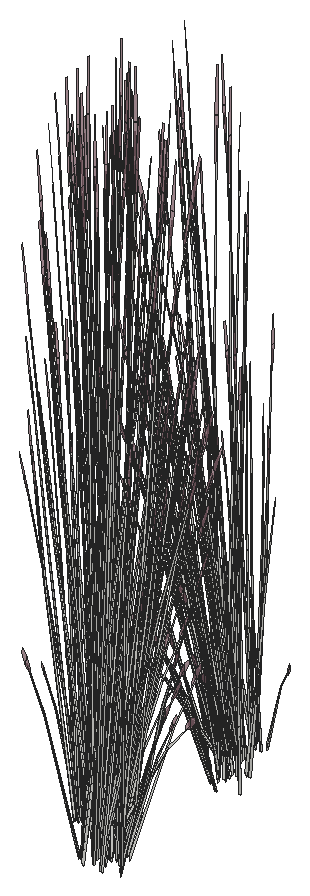
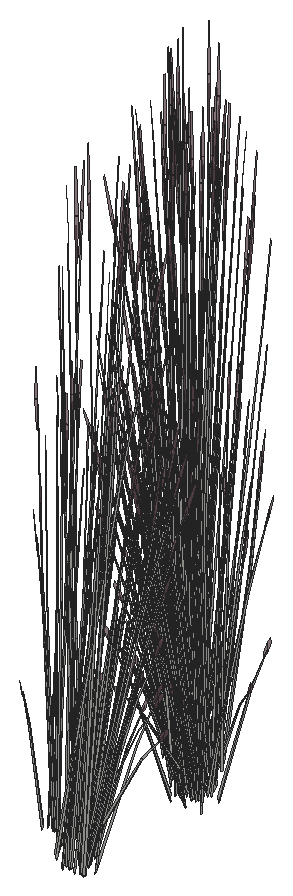
# SketchUp Ruby script. Lengths in inches.
U = 1.inch
M = Sketchup.active_model
def pt(a) = Geom::Point3d.new(a.map { |v| v * U })
def face(e, loops, mat)
  f = e.add_face(loops[0].map { |a| pt(a) })
  loops[1..].each { |l| e.add_face(l.map { |a| pt(a) }).erase! }
  f.material = f.back_material = mat if mat
  f
end
# faces: each face lists its corners as indices into pts; further lists are holes
def faces(e, pts, list, mat = nil) = list.each { |f| face(e, (f[0].is_a?(Array) ? f : [f]).map { |l| l.map { |i| pts[i] } }, mat) }
# xy, xz, yz: faces in a plane at the given z, y or x. An outline is a flat list of corners, or four numbers for a rectangle; further outlines are holes
def ring(l) = l.size == 4 ? [[l[0], l[1]], [l[2], l[1]], [l[2], l[3]], [l[0], l[3]]] : l.each_slice(2).to_a
def flat(e, list, mat, &to3) = list.each { |f| face(e, (f[0].is_a?(Array) ? f : [f]).map { |l| ring(l).map { |u, v| to3.(u, v) } }, mat) }
def xy(e, z, list, mat = nil) = flat(e, list, mat) { |x, y| [x, y, z] }
def xz(e, y, list, mat = nil) = flat(e, list, mat) { |x, z| [x, y, z] }
def yz(e, x, list, mat = nil) = flat(e, list, mat) { |y, z| [x, y, z] }
def lines(e, pts, list) = list.each { |a, b| e.add_line(pt(pts[a]), pt(pts[b])) }
# prism: a flat outline (further loops are holes) pulled along v
def prism(e, loops, v, mat = nil)
  f = face(e, loops, mat); d = Geom::Vector3d.new(v.map { |x| x * U })
  f.pushpull(f.normal.samedirection?(d) ? d.length : -d.length)
end
def box(e, o, s, mat = nil) = prism(e, [[o, [o[0] + s[0], o[1], o[2]], [o[0] + s[0], o[1] + s[1], o[2]], [o[0], o[1] + s[1], o[2]]]], [0, 0, s[2]], mat)
def at(x, y, z, deg = 0) = Geom::Transformation.translation(pt([x, y, z])) * Geom::Transformation.rotation(ORIGIN, Z_AXIS, deg.degrees)
def axes(o, x, y, z) = Geom::Transformation.new([*x, 0, *y, 0, *z, 0, *pt(o).to_a, 1])
def part(name) = M.definitions.add(name)
# library, detail: a bought-in or finely detailed component or shape, given as its bounding box
def library(name, o, s) = part(name).tap { |d| box(d.entities, o, s) }
def detail(e, o, s) = box(e.add_group.entities, o, s)
def put(e, d, t, mat = nil) = e.add_instance(d, t).tap { |i| i.material = mat if mat }
def group(e, t, mat = nil) = e.add_group.tap { |g| g.transformation = t; g.material = mat if mat }.entities
root = M.entities
M.materials.add("LightPink_Translucent").color = [144, 107, 117]
M.materials["LightPink_Translucent"].alpha = 0.75
c1 = part("blade")
p = [[2.15,0.21,22],[0,0.17,0],[0.09,0.45,0],[2.18,0.31,22],[2.29,0.31,22],[0.38,0.45,0],
  [2.48,0.24,33],[2.49,0.24,33],[2.48,0.22,33]]
faces(c1.entities,p,[[0,1,2,3],[4,5,2,3],[6,3,4,7],[8,0,3,6]])
c2 = part("seeds")
p = [[0.3,-0.1,1.38],[-0.01,-0.03,1.59],[-0.01,-0.03,0.03],[0.14,-0.07,-0.07],[0.29,-0.03,3],[0.15,0.01,3.11]]
faces(c2.entities,p,[[0,1,2,3],[1,0,4,5]],"LightPink_Translucent")
c3 = part("blade with seeds")
put(c3.entities,c1,at(0,0,0))
put(c3.entities,c2,axes([2.4,0.25,30.99],[1.5799,-0.05474,1.17369],[-0.12525,1.92788,0.29478],[-0.07173,-0.02425,1.56792]))
put(root,c3,axes([330.73,485.76,1400.21],[-0.21202,-0.39143,-0.44739],[0.32115,-0.27564,0.21531],[-0.06861,-0.04843,1.43643]))
put(root,c3,axes([330.78,485.21,1400.36],[0.15345,0.52148,0.45755],[-0.43845,0.18134,0.17955],[0.00536,-0.09582,1.58856]))
put(root,c3,axes([332.92,485.61,1399.98],[-0.22732,0.05597,1.41583],[-0.03618,-0.44548,0.08104],[0.15921,-0.06743,0.80566]))
put(root,c3,axes([333.34,485.21,1400.26],[-0.21881,-0.29821,-0.06488],[0.23965,-0.27324,-0.29416],[0.0679,-0.01924,0.97024]))
put(root,c3,axes([330.7,485.62,1400.72],[-0.17124,0.42022,0.44739],[-0.35581,-0.20224,-0.21531],[0,-0.09687,1.43643]))
put(root,c3,axes([331.33,485.25,1400.21],[0,-0.53961,0],[0.44133,0,0],[0,0,1.79456]))
put(root,c3,axes([331.87,484.01,1400.48],[-0.33032,-0.23318,0.49651],[0.19744,-0.41812,0],[0.07523,0.05311,1.57504]))
put(root,c3,axes([332.51,485.64,1402.98],[0.31014,-0.20596,-0.71045],[0.17284,0.42397,0.08574],[0.14985,-0.04816,1.00501]))
put(root,c3,axes([330.54,485.91,1400.06],[-0.36714,-0.07646,-0.62353],[0.07747,-0.47163,-0.16365],[-0.10956,-0.05715,1.37633]))
put(root,c3,axes([331.12,484.91,1400.36],[-0.29264,0.42323,0.45755],[-0.34767,-0.3736,0.17955],[0.07055,-0.04224,1.58856]))
put(root,c3,axes([331.44,485.67,1400.3],[-0.32829,-0.4014,-0.06131],[0.32849,-0.40164,0],[-0.01146,-0.01402,1.75571]))
put(root,c3,axes([330.61,484.22,1400.47],[-0.10196,0.46348,0.17642],[-0.3731,-0.13116,0.35086],[0.06445,-0.00226,1.60407]))
put(root,c3,axes([332.47,485.72,1403.05],[-0.29332,-0.1301,0.35414],[0.08555,-0.37955,-0.4572],[0.11809,-0.0348,0.87481]))
put(root,c3,axes([329.4,485.03,1402.73],[0.09971,-0.42522,0.48003],[0.32782,0.1454,0.3958],[-0.12892,0.02555,0.9933]))
put(root,c3,axes([330.46,484.59,1399.59],[-0.3474,0.18671,1.28929],[-0.11057,-0.53572,0.50096],[0.21332,0.00891,1.46642]))
put(root,c3,axes([331.39,484.73,1400.62],[0.06809,-0.4162,0.1448],[0.33266,0.07225,-0.41347],[0.06054,0.04274,1.26744]))
put(root,c3,axes([329.37,484.92,1402.73],[-0.12963,-0.31798,0.0643],[0.23638,-0.15564,0.50621],[-0.1042,0.03071,0.77189]))
put(root,c3,axes([330.82,485.72,1400.36],[0.44609,0.09826,0.45755],[-0.09078,0.55493,0.17955],[-0.06519,-0.05359,1.58856]))
put(root,c3,axes([333.17,485.32,1399.49],[-0.01845,-0.0708,1.76342],[0.12793,-0.41416,-0.26939],[0.12905,-0.00596,0.30037]))
put(root,c3,axes([329.36,485.25,1399.49],[0.00895,0.0735,1.76342],[-0.18044,0.38382,-0.26939],[-0.12817,-0.01935,0.30037]))
put(root,c3,axes([331.25,484.84,1400.72],[-0.21202,-0.39143,0.44739],[0.32115,-0.27564,-0.21531],[0.06861,0.04843,1.43643]))
put(root,c3,axes([330.15,486.63,1400.03],[-0.08291,-0.40636,-0.30978],[0.32928,-0.11539,0.30978],[-0.06638,-0.04686,1.38974]))
put(root,c3,axes([330.58,486.61,1400.47],[0.37926,-0.12378,0.17642],[0.09365,0.46065,0.35086],[-0.03382,-0.06712,1.60407]))
put(root,c3,axes([331.36,484.87,1400.67],[0.35635,-0.30962,-0.29095],[0.23697,0.43749,-0.50002],[0.08792,0.04443,1.59708]))
put(root,c3,axes([332.78,485.68,1402.53],[0.29332,0.1301,-0.35414],[-0.08555,0.37955,0.4572],[0.11809,-0.0348,0.87481]))
put(root,c3,axes([330.0625,486.8,1400.02],[-0.33032,-0.23318,-0.49651],[0.19744,-0.41812,0],[-0.07523,-0.05311,1.57504]))
put(root,c3,axes([332.26,484.04,1400.02],[0.33032,0.23318,-0.49651],[-0.19744,0.41812,0],[0.07523,0.05311,1.57504]))
put(root,c3,axes([329.33,485.08,1402.53],[-0.29332,-0.1301,-0.35414],[0.08555,-0.37955,0.4572],[-0.11809,0.0348,0.87481]))
put(root,c3,axes([331.63,485.375,1400.21],[0.39487,0,0],[0,0.48281,0],[0,0,1.78407]))
put(root,c3,axes([330.96,485.98,1400.67],[-0.35635,0.30962,-0.29095],[-0.23697,-0.43749,-0.50002],[-0.08792,-0.04443,1.59708]))
put(root,c3,axes([331.74,484.24,1400.47],[-0.37926,0.12378,0.17642],[-0.09365,-0.46065,0.35086],[0.03382,0.06712,1.60407]))
put(root,c3,axes([331.98,485.21,1401.875],[-0.14639,0.01056,1.71376],[0.09712,-0.45778,0.13857],[0.20862,0.02831,0.73262]))
put(root,c3,axes([332.17,484.22,1400.03],[0.08291,0.40636,-0.30978],[-0.32928,0.11539,0.30978],[0.06638,0.04686,1.38974]))
put(root,c3,axes([332.73,485.84,1402.73],[0.12963,0.31798,0.0643],[-0.23638,0.15564,0.50621],[0.1042,-0.03071,0.77189]))
put(root,c3,axes([331.5,485.13,1400.38],[-0.44609,-0.09826,0.49198],[0.09078,-0.55493,0.19306],[0.06519,0.05359,1.70813]))
put(root,c3,axes([332.71,485.73,1402.73],[-0.09971,0.42522,0.48003],[-0.32782,-0.1454,0.3958],[0.12892,-0.02555,0.9933]))
put(root,c3,axes([331.15,486.5,1400.2],[-0.11516,-0.40207,0],[0.32884,-0.1408,0],[0,0,1.54371]))
put(root,c3,axes([330.93,486.12,1400.62],[-0.06809,0.4162,0.1448],[-0.33266,-0.07225,-0.41347],[-0.06054,-0.04274,1.26744]))
put(root,c3,axes([329.64,485.04,1403.05],[0.29332,0.1301,0.35414],[-0.08555,0.37955,-0.4572],[-0.11809,0.0348,0.87481]))
put(root,c3,axes([331.58,486.44,1400.18],[0.37054,-0.15823,-0.19198],[0.1302,0.45581,0.00008],[0.0409,-0.01749,1.73897]))
put(root,c3,axes([331.71,486.63,1400.47],[0.10196,-0.46348,0.17642],[0.3731,0.13116,0.35086],[-0.06445,0.00226,1.60407]))
put(root,c3,axes([331.62,485.58,1400.21],[0.24637,0.30123,0],[-0.24637,0.30123,0],[0,0,1.69266]))
put(root,c3,axes([330.22,485.01,1401.34],[0.10032,-0.06746,1.77064],[0.0346,0.47103,0.13857],[-0.2173,0.0625,0.63284]))
put(root,c3,axes([332.29,485.45,1400.47],[-0.2773,-0.3397,0.17642],[0.27945,-0.32949,0.35086],[-0.03063,0.06937,1.60407]))
put(root,c3,axes([331.78,484.9375,1400.06],[0.36714,0.07646,-0.62353],[-0.07747,0.47163,-0.16365],[0.10956,0.05715,1.37633]))
put(root,c3,axes([333.4,485.76,1400.77],[-0.21807,0.07699,1.1486],[0.10265,-0.31819,0.84392],[0.11568,0.02177,0.25299]))
put(root,c3,axes([331.07,486.68,1400.2],[-0.35581,-0.20937,0],[0.17124,-0.43505,0],[0,0,1.62707]))
put(root,c3,axes([331.36,486.12,1400.46],[-0.34464,-0.37536,-0.25192],[0.29,-0.42149,0.5513],[-0.0928,0.04391,1.68216]))
put(root,c3,axes([330.45,486.84,1400.48],[0.33032,0.23318,0.49651],[-0.19744,0.41812,0],[-0.07523,-0.05311,1.57504]))
put(root,c3,axes([331.62,485.23,1400.72],[0.17124,-0.42022,0.44739],[0.35581,0.20224,-0.21531],[0,0.09687,1.43643]))
put(root,c3,axes([333.3,487.11,1402.71],[-0.03191,-0.04083,1.77383],[0.06981,-0.43764,-0.16761],[0.12571,-0.02796,0.31391]))
put(root,c3,axes([329.14,485.33,1402.72],[-0.05763,0.06055,1.74944],[0.0049,0.44239,-0.27667],[-0.13211,0.05753,0.14031]))
put(root,c3,axes([331.55,485.47,1400.29],[0,0.53934,-0.05637],[-0.44133,0,0],[0,0.01695,1.79368]))
put(root,c3,axes([329.53,485.27,1402.68],[-0.09562,0.42421,-0.51099],[-0.32782,-0.1454,-0.3958],[-0.13199,0.0389,0.97773]))
put(root,c3,axes([329.51,484.91,1403.03],[0.17758,0.42229,-0.1216],[-0.31518,0.20752,-0.67495],[-0.13282,0.05572,1.02557]))
put(root,c3,axes([331.58,485.09,1400.21],[0.21202,0.39143,-0.44739],[-0.32115,0.27564,0.21531],[0.06861,0.04843,1.43643]))
put(root,c3,axes([333.02,486.74,1401.93],[-0.06755,-0.39203,-0.03492],[0.31928,-0.09013,-0.15832],[0.06667,0.02485,0.52218]))
put(root,c3,axes([330.26,487.09,1400.375],[-0.22066,0.46731,0],[-0.36918,-0.26061,-0.51607],[-0.08408,-0.05936,1.63711]))
put(root,c3,axes([332.19,486.73,1403.03],[0.0189,-0.47427,-0.1216],[0.35781,0.01296,-0.67495],[0.13781,0.03295,1.02557]))
put(root,c3,axes([332.52,485.46,1400.48],[0,-0.46636,0.49651],[0.39487,0,0],[0,0.10622,1.57504]))
put(root,c3,axes([331.53,485.8125,1400.72],[0.38326,-0.02879,0.44739],[0.03466,0.47788,-0.21531],[-0.06861,0.04843,1.43643]))
put(root,c3,axes([331.77,485.32,1400.62],[0.32884,-0.136,0.1448],[0.11516,0.38837,-0.41347],[0,0.08547,1.26744]))
put(root,c3,axes([332.14,486.54,1403.05],[-0.20082,-0.29199,0.35414],[0.2293,-0.2764,-0.4572],[0.1165,0.04206,0.87481]))
put(root,c3,axes([331.1875,486.04,1400.21],[-0.38326,0.02879,-0.44739],[-0.03466,-0.47788,0.21531],[-0.06861,0.04843,1.43643]))
put(root,c3,axes([332.99,486.27,1400.59],[-0.085,-0.1147,1.43002],[0.1106,-0.37943,-0.30754],[0.17198,0.0514,0.61141]))
put(root,c3,axes([331.47,486.6875,1400.2],[0.35581,0.20937,0],[-0.17124,0.43505,0],[0,0,1.74954]))
put(root,c3,axes([332.5,486.44,1402.72],[0.07571,-0.00789,1.74944],[0.20767,-0.36231,-0.27667],[0.13467,0.04783,0.14031]))
put(root,c3,axes([331.61,487.15,1400.19],[-0.21791,-0.46895,-0.05142],[0.36918,-0.26061,0.51607],[-0.09097,0.04465,1.6363]))
put(root,c3,axes([331.53,486.02,1400.62],[0.26075,0.2802,0.1448],[-0.2175,0.31612,-0.41347],[-0.06054,0.04274,1.26744]))
put(root,c3,axes([329.47,486.09,1402.73],[-0.08753,-0.42921,0.48003],[0.34336,-0.07449,0.3958],[-0.1012,0.10094,0.9933]))
put(root,c3,axes([329.41,486.01,1402.73],[-0.2423,-0.19613,0.0643],[0.14107,-0.2793,0.50621],[-0.07768,0.0903,0.77189]))
put(root,c3,axes([329.52,485.49,1401.875],[0.12246,-0.09864,1.71376],[0.1031,0.45582,0.13857],[-0.19225,0.10302,0.73262]))
put(root,c3,axes([332.21,486.5,1402.98],[0.35281,0.01123,-0.71045],[-0.0237,0.47284,0.08574],[0.14947,0.0499,1.00501]))
put(root,c3,axes([331.8125,486.88,1400.48],[0.33032,-0.23318,0.49651],[0.19744,0.41812,0],[-0.07523,0.05311,1.57504]))
put(root,c3,axes([331.34,486.51,1400.29],[0.15345,0.53576,-0.06012],[-0.43845,0.18773,0],[0.00536,0.01871,1.72173]))
put(root,c3,axes([331.51,487.09,1400.03],[-0.32928,-0.11539,-0.30978],[0.08291,-0.40636,0.30978],[-0.06638,0.04686,1.38974]))
put(root,c3,axes([329.14,486.27,1400.59],[0.12266,0.03828,1.43002],[0.07906,0.39104,-0.30754],[-0.16661,0.0732,0.61141]))
put(root,c3,axes([329.6875,485.95,1403.05],[0.30722,-0.06665,0.35414],[0.08112,0.381,-0.4572],[-0.08804,0.10234,0.87481]))
put(root,c3,axes([332.78,485.54,1400.375],[0.44133,0,0],[0,0.52122,-0.51607],[0,0.11871,1.63711]))
put(root,c3,axes([328.5,485.78,1402.71],[0.04504,0.01251,1.77383],[0.13934,0.41205,-0.16761],[-0.0922,0.10815,0.31391]))
put(root,c3,axes([332.61,485.81,1400.2],[-0.44111,-0.00373,-0.04976],[0,-0.52122,0.49943],[-0.01386,0.11865,1.58352]))
put(root,c3,axes([331.65,485.36,1400.67],[0.39748,0.22252,-0.29095],[-0.19139,0.46966,-0.50002],[0.01249,0.11531,1.59708]))
put(root,c3,axes([328.88,487.09,1400.77],[0.14709,-0.21136,1.1486],[0.05804,0.3346,0.84392],[-0.1063,0.05991,0.25299]))
put(root,c3,axes([332.42,486.7,1402.53],[0.20082,0.29199,-0.35414],[-0.2293,0.2764,0.4572],[0.1165,0.04206,0.87481]))
put(root,c3,axes([332.52,485.89,1400.03],[-0.24637,0.29097,-0.30978],[-0.24637,-0.29097,0.30978],[0,0.09372,1.38974]))
put(root,c3,axes([331.46,485.91,1400.67],[0.04113,0.53214,-0.29095],[-0.42835,0.03218,-0.50002],[-0.07543,0.07088,1.59708]))
put(root,c3,axes([332.32,486.81,1402.73],[-0.01777,0.35463,0.0643],[-0.26836,-0.00972,0.50621],[0.1028,0.03711,0.77189]))
put(root,c3,axes([331.61,485.71,1400.21],[-0.17124,0.42022,-0.44739],[-0.35581,-0.20224,0.21531],[0,0.09687,1.43643]))
put(root,c3,axes([329.43,486.17,1402.53],[-0.30722,0.06665,-0.35414],[-0.08112,-0.381,0.4572],[-0.08804,0.10234,0.87481]))
put(root,c3,axes([332.34,486.7,1402.73],[-0.26024,0.30729,0.48003],[-0.22444,-0.32634,0.3958],[0.1221,0.05668,0.9933]))
put(root,c3,axes([328.99,487.03,1403.65],[0.31145,0.12449,-0.06488],[-0.0958,0.38314,-0.29416],[-0.05094,0.05817,0.97024]))
put(root,c3,axes([331.2,486.32,1400.06],[-0.23773,0.35053,-0.62353],[-0.29532,-0.31785,-0.16365],[-0.09526,0.08744,1.37633]))
put(root,c3,axes([331.52,487.05,1403.05],[-0.05451,-0.37564,0.35414],[0.31161,-0.09919,-0.4572],[0.0837,0.10765,0.87481]))
put(root,c3,axes([331.62,486.91,1400.33],[0.44186,0.15158,0.30756],[-0.11054,0.54181,-0.36492],[-0.07313,0.06781,1.64885]))
put(root,c3,axes([331.59,487.28,1400.02],[-0.33032,0.23318,-0.49651],[-0.19744,-0.41812,0],[-0.07523,0.05311,1.57504]))
put(root,c3,axes([332.6875,485.9,1400.02],[0,0.46636,-0.49651],[-0.39487,0,0],[0,0.10622,1.57504]))
put(root,c3,axes([331.7,485.95,1401.875],[-0.1311,-0.08035,1.71376],[0.27131,-0.33708,0.13857],[0.16909,0.15206,0.73262]))
put(root,c3,axes([331.72,484.89,1402.47],[-0.30498,-0.24231,1.38283],[0.32203,-0.37727,0.59665],[0.0984,0.22736,1.33663]))
put(root,c3,axes([329.53,485.91,1403.03],[0.32648,0.25715,-0.1216],[-0.18809,0.3724,-0.67495],[-0.09224,0.12945,1.02557]))
put(root,c3,axes([332.18,486.86,1400.77],[-0.19872,-0.13409,1.1486],[0.2566,-0.13625,0.84392],[0.06921,0.11541,0.25299]))
put(root,c3,axes([331.49,487.25,1403.03],[0.21031,-0.39918,-0.1216],[0.30457,0.22997,-0.67495],[0.10587,0.11278,1.02557]))
put(root,c3,axes([329.97,485.8,1401.875],[0.08815,-0.14329,1.71376],[0.22258,0.38678,0.13857],[-0.15267,0.17614,0.73262]))
put(root,c3,axes([329.6875,486.22,1402.68],[0.09067,0.42583,-0.51099],[-0.34336,0.07449,-0.3958],[-0.0984,0.11438,0.97773]))
put(root,c3,axes([330.1,486.71,1403.05],[0.23881,-0.24554,0.35414],[0.22606,0.28036,-0.4572],[-0.0344,0.14245,0.87481]))
put(root,c3,axes([331.89,487.2,1400.375],[0.22066,0.46731,0],[-0.36918,0.26061,-0.51607],[-0.08408,0.05936,1.63711]))
put(root,c3,axes([331.21,487.58,1402.71],[0.00104,-0.05646,1.77383],[0.30246,-0.2491,-0.16761],[0.10506,0.08891,0.31391]))
put(root,c3,axes([332.24,487.36,1399.49],[0.02571,-0.06733,1.76342],[0.32373,-0.19829,-0.26939],[0.09815,0.10263,0.30037]))
put(root,c3,axes([331.7,485.35,1400.84],[-0.00964,-0.43909,1.41272],[0.43635,0.11382,0.59816],[-0.1032,0.24027,1.3335]))
put(root,c3,axes([331.8125,485.83,1400.09],[0.12941,0.42699,-0.69212],[-0.37279,0.15378,-0.18165],[0.0143,0.14459,1.52773]))
put(root,c3,axes([329.88,486.93,1402.73],[-0.29004,-0.02173,0.0643],[0.00795,-0.32812,0.50621],[-0.03035,0.12569,0.77189]))
put(root,c3,axes([329.27,487.3,1399.49],[0.04734,0.04659,1.76342],[0.08027,0.4317,-0.26939],[-0.10492,0.09206,0.30037]))
put(root,c3,axes([329.98,486.96,1402.73],[-0.25132,-0.3182,0.48003],[0.2669,-0.27442,0.3958],[-0.04636,0.14929,0.9933]))
put(root,c3,axes([331.74,487.05,1402.68],[0.34827,-0.11086,-0.51099],[0.06092,0.41983,-0.3958],[0.09354,0.12031,0.97773]))
put(root,c3,axes([330.77,487.11,1403.05],[0.1064,-0.35863,0.35414],[0.31043,0.1046,-0.4572],[0.02846,0.14439,0.87481]))
put(root,c3,axes([332.22,487.47,1400.67],[-0.22633,-0.01463,1.0506],[0.14947,-0.31064,0.58006],[0.08941,0.11036,0.8241]))
put(root,c3,axes([331.56,487.39,1402.73],[-0.16041,0.29625,0.0643],[-0.22843,-0.17248,0.50621],[0.07385,0.09498,0.77189]))
put(root,c3,axes([331.1875,488.39,1403.65],[0.2439,-0.26754,-0.06488],[0.22348,0.29302,-0.29416],[0.01573,0.08303,0.97024]))
put(root,c3,axes([331.63,487.31,1402.73],[-0.35104,0.10702,0.48003],[-0.06092,-0.41983,0.3958],[0.08256,0.12373,0.9933]))
put(root,c3,axes([329.9,486.15,1401.875],[0.06572,-0.16029,1.71376],[0.27569,0.33172,0.13857],[-0.12437,0.20675,0.73262]))
put(root,c3,axes([331.48,486.72,1400.59],[0.00623,-0.15459,1.43002],[0.29764,-0.17268,-0.30754],[0.09188,0.18503,0.61141]))
put(root,c3,axes([330.67,487.44,1402.73],[-0.26007,0.1585,0.0643],[-0.12729,-0.28902,0.50621],[0.02512,0.1274,0.77189]))
put(root,c3,axes([329.98,487.05,1402.53],[-0.23881,0.24554,-0.35414],[-0.22606,-0.28036,0.4572],[-0.0344,0.14245,0.87481]))
put(root,c3,axes([329.15,486.98,1402.72],[-0.00877,0.09229,1.74944],[0.24897,0.32105,-0.27667],[-0.06518,0.15182,0.14031]))
put(root,c3,axes([329.95,486.77,1403.4],[0.3879,0.02311,-0.13498],[-0.0106,0.43749,-0.74919],[-0.02694,0.1685,1.13838]))
put(root,c3,axes([330.67,487.26,1403.03],[0.34538,-0.21713,-0.1216],[0.16972,0.38536,-0.67495],[0.04557,0.16239,1.02557]))
put(root,c3,axes([330.77,487.4,1403.0625],[-0.34777,-0.12192,0.53283],[0.11892,-0.40083,0.43934],[0.0209,0.15763,1.10256]))
put(root,c3,axes([330.13,488.01,1400.77],[-0.00913,-0.2773,1.1486],[0.22824,0.19778,0.84392],[-0.04489,0.13217,0.25299]))
put(root,c3,axes([330.73,487.35,1399.49],[0.05712,-0.02538,1.76342],[0.34359,0.13968,-0.26939],[0.01005,0.15742,0.30037]))
put(root,c3,axes([330.21,486.9375,1403],[0.25266,0.31335,-0.5672],[-0.2669,0.27442,-0.43934],[-0.03844,0.15921,1.08528]))
put(root,c3,axes([329.9375,487.41,1400.82],[0.32063,-0.08258,0.06507],[0.07371,0.33271,-0.86304],[-0.02033,0.16842,0.7736]))
put(root,c3,axes([330.96,487.24,1402.68],[0.34695,0.11691,-0.51099],[-0.11892,0.40083,-0.3958],[0.03181,0.16138,0.97773]))
put(root,c3,axes([331.16,486.41,1401.875],[-0.08068,-0.14973,1.71376],[0.3728,-0.12606,0.13857],[0.08426,0.23506,0.73262]))
put(root,c3,axes([330.8,487.49,1402.53],[-0.1064,0.35863,-0.35414],[-0.31043,-0.1046,0.4572],[0.02846,0.14439,0.87481]))
put(root,c3,axes([330.13,486.8,1403.34],[-0.00918,0.43138,-0.7886],[-0.38672,-0.02897,0.09517],[-0.04081,0.18275,1.11556]))
put(root,c3,axes([329.125,487.93,1402.71],[0.04004,-0.02816,1.77383],[0.33095,0.18728,-0.16761],[-0.00778,0.15594,0.31391]))
put(root,c3,axes([330.5,486.49,1401.875],[-0.00864,-0.17899,1.71376],[0.37441,0.11874,0.13857],[-0.02316,0.25508,0.73262]))
put(root,c3,axes([330.84,487.17,1402.98],[0.16845,0.3792,-0.71045],[-0.34676,0.21133,0.08574],[0.03939,0.18322,1.00501]))
put(root,c3,axes([329.86,487.76,1400.59],[0.11138,-0.07357,1.43002],[0.27499,0.22183,-0.30754],[-0.08185,0.19194,0.61141]))
put(root,c3,axes([330.58,488.125,1402.72],[0.04474,0.0751,1.74944],[0.36104,0.0295,-0.27667],[0.03631,0.16562,0.14031]))
put(root,c3,axes([330.01,487.4,1401.36],[0.00775,-0.24075,1.54345],[0.34877,0.12716,0.21329],[-0.03022,0.25658,0.72882]))
put(root,c3,axes([330.27,499.5,1401.875],[0.08068,0.14973,1.71376],[-0.3728,0.12606,0.13857],[-0.08426,-0.23506,0.73262]))
put(root,c3,axes([330.89,498.51,1402.72],[-0.05398,-0.06539,1.74944],[-0.36026,0.04145,-0.27667],[-0.0575,-0.15639,0.14031]))
put(root,c3,axes([331.72,499.28,1400.59],[-0.10032,0.0944,1.43002],[-0.30046,-0.16522,-0.30754],[0.05569,-0.20547,0.61141]))
put(root,c3,axes([331.27,499.61,1402.98],[-0.16845,-0.3792,-0.71045],[0.34676,-0.21133,0.08574],[-0.03939,-0.18322,1.00501]))
put(root,c3,axes([330.17,499.11,1400.59],[-0.02137,0.15256,1.43002],[-0.31245,0.12771,-0.30754],[-0.07303,-0.19719,0.61141]))
put(root,c3,axes([330.98,498.77,1399.49],[-0.0592,0.0168,1.76342],[-0.32738,-0.18913,-0.26939],[0.00549,-0.15776,0.30037]))
put(root,c3,axes([331.97,499.98,1402.98],[0.00918,-0.43138,-0.71045],[0.38672,0.02897,0.08574],[0.04081,-0.18275,1.00501]))
put(root,c3,axes([332.51,499.31,1402.72],[-0.00341,-0.09282,1.74944],[-0.28775,-0.26825,-0.27667],[0.04449,-0.16261,0.14031]))
put(root,c3,axes([331.3,499.29,1402.53],[0.1064,-0.35863,-0.35414],[0.31043,0.1046,0.4572],[-0.02846,-0.14439,0.87481]))
put(root,c3,axes([331.53,499.76,1401.875],[-0.06572,0.16029,1.71376],[-0.27569,-0.33172,0.13857],[0.12437,-0.20675,0.73262]))
put(root,c3,axes([332.43,498.98,1402.71],[-0.03584,0.03562,1.77383],[-0.35118,-0.12018,-0.16761],[-0.01271,-0.15545,0.31391]))
put(root,c3,axes([331.14,499.54,1402.68],[-0.34695,-0.11691,-0.51099],[0.11892,-0.40083,-0.3958],[-0.03181,-0.16138,0.97773]))
put(root,c3,axes([331.35,498.53,1400.77],[0.04528,0.27194,1.1486],[-0.25117,-0.15062,0.84392],[0.02703,-0.13924,0.25299]))
put(root,c3,axes([331.89,499.84,1402.68],[-0.25266,-0.31335,-0.51099],[0.2669,-0.27442,-0.3958],[0.03844,-0.15921,0.97773]))
put(root,c3,axes([330.52,498.29,1402.71],[-0.00658,0.0559,1.77383],[-0.32474,0.20287,-0.16761],[-0.09556,-0.1037,0.31391]))
put(root,c3,axes([330.45,499.29,1403.09],[0.39316,-0.11987,0.53763],[0.06823,0.47021,0.4433],[-0.09247,-0.13858,1.11249]))
put(root,c3,axes([331.34,499.375,1402.73],[0.34777,0.12192,0.48003],[-0.11892,0.40083,0.3958],[-0.0209,-0.15763,0.9933]))
put(root,c3,axes([331.4375,499.52,1403.03],[-0.34538,0.21713,-0.1216],[-0.16972,-0.38536,-0.67495],[-0.04557,-0.16239,1.02557]))
put(root,c3,axes([332.15,500,1403.03],[-0.3879,-0.02311,-0.1216],[0.0106,-0.43749,-0.67495],[0.02694,-0.1685,1.02557]))
put(root,c3,axes([332.13,499.72,1402.53],[0.23881,-0.24554,-0.35414],[0.22606,0.28036,0.4572],[0.0344,-0.14245,0.87481]))
put(root,c3,axes([330.0625,498.86,1400.77],[0.18411,0.16231,1.1486],[-0.26813,0.09757,0.84392],[-0.05737,-0.12474,0.25299]))
put(root,c3,axes([331.43,499.34,1402.73],[0.26007,-0.1585,0.0643],[0.12729,0.28902,0.50621],[-0.02512,-0.1274,0.77189]))
put(root,c3,axes([330.51,499.72,1402.98],[-0.30095,-0.22541,-0.71045],[0.21388,-0.395,0.08574],[-0.10904,-0.13459,1.00501]))
put(root,c3,axes([330.4,499.42,1402.53],[-0.05451,-0.37564,-0.35414],[0.31161,-0.09919,0.4572],[-0.0837,-0.10765,0.87481]))
put(root,c3,axes([330.54,499.39,1402.73],[0.16041,-0.29625,0.0643],[0.22843,0.17248,0.50621],[-0.07385,-0.09498,0.77189]))
put(root,c3,axes([329.92,499.35,1399.49],[-0.03419,0.06144,1.76342],[-0.3455,0.13246,-0.26939],[-0.08346,-0.12049,0.30037]))
put(root,c3,axes([330.49,501.04,1400.1],[-0.14494,-0.47823,-0.69835],[0.41752,-0.17223,-0.18329],[-0.01602,-0.16194,1.54149]))
put(root,c3,axes([329.73,499.97,1401.875],[0.1311,0.08035,1.71376],[-0.27131,0.33708,0.13857],[-0.16909,-0.15206,0.73262]))
put(root,c3,axes([332.43,499.58,1399.49],[-0.05283,-0.03674,1.76342],[-0.13569,-0.41045,-0.26939],[0.09154,-0.11138,0.30037]))
put(root,c3,axes([331.33,499.67,1403.05],[-0.1064,0.35863,0.35414],[-0.31043,-0.1046,-0.4572],[-0.02846,-0.14439,0.87481]))
put(root,c3,axes([330.37,499.73,1402.68],[-0.34827,0.11086,-0.51099],[-0.06092,-0.41983,-0.3958],[-0.09354,-0.12031,0.97773]))
put(root,c3,axes([332.125,499.82,1402.73],[0.25132,0.3182,0.48003],[-0.2669,0.27442,0.3958],[0.04636,-0.14929,0.9933]))
put(root,c3,axes([330.61,499.36,1403.43],[-0.23555,0.44708,-0.13619],[-0.34112,-0.25757,-0.75594],[-0.11858,-0.12631,1.14864]))
put(root,c3,axes([332.22,499.85,1402.73],[0.29004,0.02173,0.0643],[-0.00795,0.32812,0.50621],[0.03035,-0.12569,0.77189]))
put(root,c3,axes([332,500.07,1403.05],[-0.23881,0.24554,0.35414],[-0.22606,-0.28036,-0.4572],[0.0344,-0.14245,0.87481]))
put(root,c3,axes([332.42,500.73,1402.98],[0.18436,-0.36797,-0.71045],[0.32306,0.26151,0.08574],[0.11008,-0.13332,1.00501]))
put(root,c3,axes([330.43,499.66,1400.375],[-0.22066,-0.46731,0],[0.36918,-0.26061,-0.51607],[0.08408,-0.05936,1.63711]))
put(root,c3,axes([332.41,500.5625,1402.68],[-0.09067,-0.42583,-0.51099],[0.34336,-0.07449,-0.3958],[0.0984,-0.11438,0.97773]))
put(root,c3,axes([330.92,499.1,1400.13],[-0.2439,0.26754,-0.03893],[-0.22348,-0.29302,-0.17649],[-0.01573,-0.08303,0.58215]))
put(root,c3,axes([329.71,499.23,1402.72],[-0.07594,-0.00329,1.74944],[-0.24177,0.32918,-0.27667],[-0.129,-0.06726,0.14031]))
put(root,c3,axes([332.58,500.87,1403.03],[-0.32648,-0.25715,-0.1216],[0.18809,-0.3724,-0.67495],[0.09224,-0.12945,1.02557]))
put(root,c3,axes([331.23,502.27,1401.33],[0.305,0.18805,1.51261],[-0.29879,0.40513,0.59816],[-0.13384,-0.24012,1.26806]))
put(root,c3,axes([330.59,499.73,1403.05],[0.05451,0.37564,0.35414],[-0.31161,0.09919,-0.4572],[-0.0837,-0.10765,0.87481]))
put(root,c3,axes([329.63,500.97,1400.02],[0,-0.46636,-0.49651],[0.39487,0,0],[0,-0.10622,1.57504]))
put(root,c3,axes([330.73,499.59,1400.02],[0.33032,-0.23318,-0.49651],[0.19744,0.41812,0],[0.07523,-0.05311,1.57504]))
put(root,c3,axes([332.69,500.39,1400.59],[-0.12609,-0.01381,1.43002],[-0.12917,-0.37055,-0.30754],[0.1549,-0.10482,0.61141]))
put(root,c3,axes([329.65,499.97,1403.09],[0.29147,-0.34417,0.53763],[0.25138,0.3655,0.4433],[-0.13675,-0.06349,1.11249]))
put(root,c3,axes([333.38,500.75,1402.71],[-0.0461,-0.00354,1.77383],[-0.19143,-0.37951,-0.16761],[0.07688,-0.12478,0.31391]))
put(root,c3,axes([331.12,500.55,1400.06],[0.23773,-0.35053,-0.62353],[0.29532,0.31785,-0.16365],[0.09526,-0.08744,1.37633]))
put(root,c3,axes([332.84,499.71,1400.77],[-0.11756,0.2374,1.1486],[-0.10105,-0.31895,0.84392],[0.09709,-0.07992,0.25299]))
put(root,c3,axes([332.67,500.61,1402.53],[0.30722,-0.06665,-0.35414],[0.08112,0.381,0.4572],[0.08804,-0.10234,0.87481]))
put(root,c3,axes([329.78,499.97,1402.73],[0.01777,-0.35463,0.0643],[0.26836,0.00972,0.50621],[-0.1028,-0.03711,0.77189]))
put(root,c3,axes([330.71,501.16,1400.21],[0.17124,-0.42022,-0.44739],[0.35581,0.20224,0.21531],[0,-0.09687,1.43643]))
put(root,c3,axes([329.68,500.08,1402.53],[-0.20082,-0.29199,-0.35414],[0.2293,-0.2764,0.4572],[-0.1165,-0.04206,0.87481]))
put(root,c3,axes([330.86,500.95,1400.67],[-0.04113,-0.53214,-0.29095],[0.42835,-0.03218,-0.50002],[0.07543,-0.07088,1.59708]))
put(root,c3,axes([329.8,500.98,1400.03],[0.24637,-0.29097,-0.30978],[0.24637,0.29097,0.30978],[0,-0.09372,1.38974]))
put(root,c3,axes([329.7,499.58,1400.13],[-0.10181,0.3808,-0.03893],[-0.31336,-0.11714,-0.17649],[-0.04758,-0.06228,0.58215]))
put(root,c3,axes([332.42,500.83,1403.05],[-0.30722,0.06665,0.35414],[-0.08112,-0.381,-0.4572],[0.08804,-0.10234,0.87481]))
put(root,c3,axes([330.67,501.51,1400.67],[-0.39748,-0.22252,-0.29095],[0.19139,-0.46966,-0.50002],[-0.01249,-0.11531,1.59708]))
put(root,c3,axes([329.53,501.32,1400.375],[-0.44133,0,0],[0,-0.52122,-0.51607],[0,-0.11871,1.63711]))
put(root,c3,axes([329.61,500.39,1400.59],[0.06891,0.12984,1.43002],[-0.15879,0.35293,-0.30754],[-0.16304,-0.08436,0.61141]))
put(root,c3,axes([330.81,499.77,1400.03],[0.32928,0.11539,-0.30978],[-0.08291,0.40636,0.30978],[0.06638,-0.04686,1.38974]))
put(root,c3,axes([329.89,500.28,1402.98],[-0.35281,-0.01123,-0.71045],[0.0237,-0.47284,0.08574],[-0.14947,-0.0499,1.00501]))
put(root,c3,axes([332.7,500.77,1402.73],[0.2423,0.19613,0.0643],[-0.14107,0.2793,0.50621],[0.07768,-0.0903,0.77189]))
put(root,c3,axes([332.63,500.6875,1402.73],[0.08753,0.42921,0.48003],[-0.34336,0.07449,0.3958],[0.1012,-0.10094,0.9933]))
put(root,c3,axes([333.55,501.21,1402.72],[0.04898,-0.07104,1.74944],[-0.06269,-0.43574,-0.27667],[0.12289,-0.08262,0.14031]))
put(root,c3,axes([329.875,501.1875,1400.33],[-0.32829,0.39208,0.30756],[-0.32849,-0.38796,-0.36492],[-0.01146,-0.11134,1.64885]))
put(root,c3,axes([329.42,499.51,1402.71],[0.02617,0.04654,1.77383],[-0.12614,0.41836,-0.16761],[-0.12775,0.00303,0.31391]))
put(root,c3,axes([330.92,501.37,1400.43],[0.39767,0.22603,0.24065],[-0.19139,0.46966,0.50002],[0,-0.10827,1.60543]))
put(root,c3,axes([330.77,502,1400.4375],[0.09355,-0.55261,-0.23429],[0.44354,0.09633,0.51271],[-0.0775,-0.07631,1.5644]))
